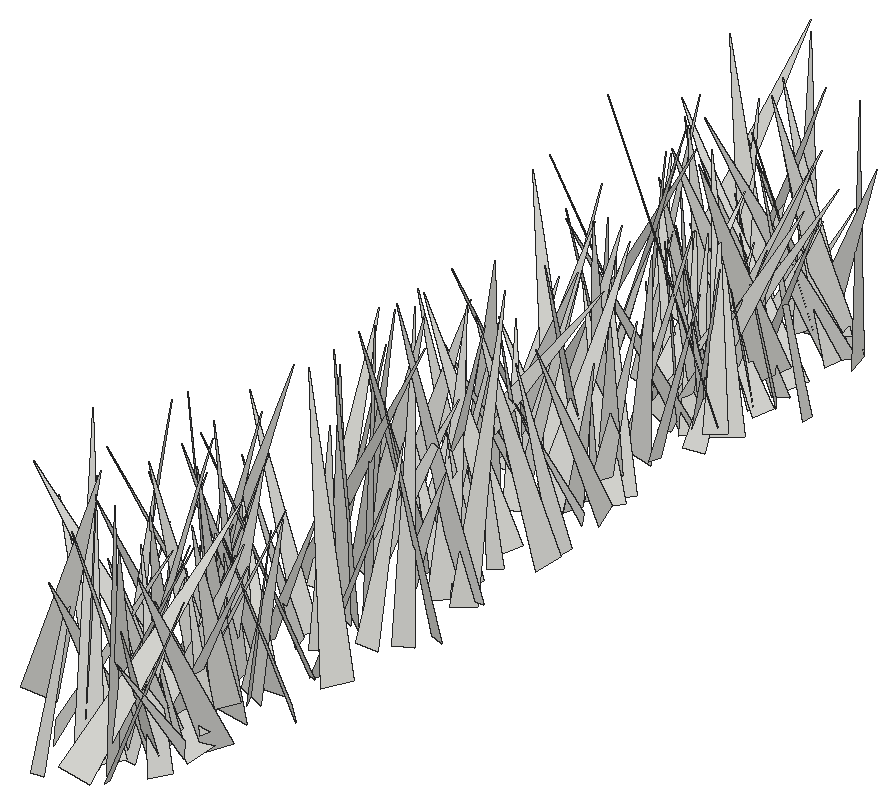
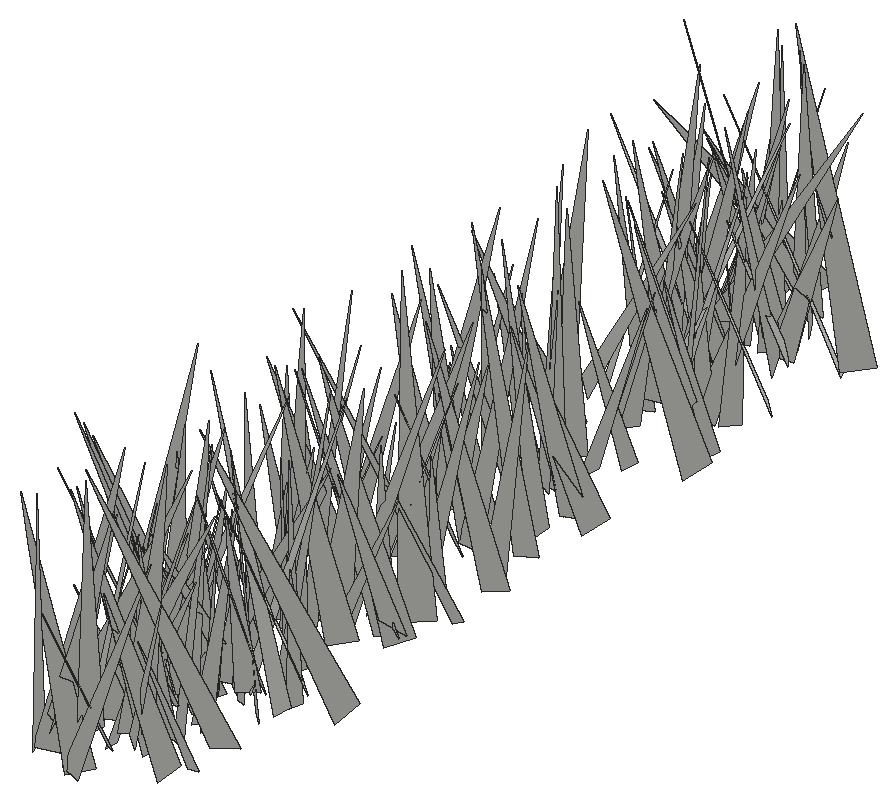
# SketchUp Ruby script. Lengths in inches.
U = 1.inch
M = Sketchup.active_model
def pt(a) = Geom::Point3d.new(a.map { |v| v * U })
def face(e, loops, mat)
  f = e.add_face(loops[0].map { |a| pt(a) })
  loops[1..].each { |l| e.add_face(l.map { |a| pt(a) }).erase! }
  f.material = f.back_material = mat if mat
  f
end
# faces: each face lists its corners as indices into pts; further lists are holes
def faces(e, pts, list, mat = nil) = list.each { |f| face(e, (f[0].is_a?(Array) ? f : [f]).map { |l| l.map { |i| pts[i] } }, mat) }
# xy, xz, yz: faces in a plane at the given z, y or x. An outline is a flat list of corners, or four numbers for a rectangle; further outlines are holes
def ring(l) = l.size == 4 ? [[l[0], l[1]], [l[2], l[1]], [l[2], l[3]], [l[0], l[3]]] : l.each_slice(2).to_a
def flat(e, list, mat, &to3) = list.each { |f| face(e, (f[0].is_a?(Array) ? f : [f]).map { |l| ring(l).map { |u, v| to3.(u, v) } }, mat) }
def xy(e, z, list, mat = nil) = flat(e, list, mat) { |x, y| [x, y, z] }
def xz(e, y, list, mat = nil) = flat(e, list, mat) { |x, z| [x, y, z] }
def yz(e, x, list, mat = nil) = flat(e, list, mat) { |y, z| [x, y, z] }
def lines(e, pts, list) = list.each { |a, b| e.add_line(pt(pts[a]), pt(pts[b])) }
# prism: a flat outline (further loops are holes) pulled along v
def prism(e, loops, v, mat = nil)
  f = face(e, loops, mat); d = Geom::Vector3d.new(v.map { |x| x * U })
  f.pushpull(f.normal.samedirection?(d) ? d.length : -d.length)
end
def box(e, o, s, mat = nil) = prism(e, [[o, [o[0] + s[0], o[1], o[2]], [o[0] + s[0], o[1] + s[1], o[2]], [o[0], o[1] + s[1], o[2]]]], [0, 0, s[2]], mat)
def at(x, y, z, deg = 0) = Geom::Transformation.translation(pt([x, y, z])) * Geom::Transformation.rotation(ORIGIN, Z_AXIS, deg.degrees)
def axes(o, x, y, z) = Geom::Transformation.new([*x, 0, *y, 0, *z, 0, *pt(o).to_a, 1])
def part(name) = M.definitions.add(name)
# library, detail: a bought-in or finely detailed component or shape, given as its bounding box
def library(name, o, s) = part(name).tap { |d| box(d.entities, o, s) }
def detail(e, o, s) = box(e.add_group.entities, o, s)
def put(e, d, t, mat = nil) = e.add_instance(d, t).tap { |i| i.material = mat if mat }
def group(e, t, mat = nil) = e.add_group.tap { |g| g.transformation = t; g.material = mat if mat }.entities
root = M.entities
c1 = part("fur_instance\#9")
p = [[0.8125,0,1.79],[0.67,-0.02,1.48],[0,-0.11,0],[0,0.11,0]]
faces(c1.entities,p,[[0,1,2,3]])
put(root,c1,axes([152.47,140.48,-27.1],[5.88559,1.89129,2.87248],[1.95642,-6.52369,0.2867],[-2.82853,-0.57687,6.17535]))
put(root,c1,axes([150.89,143.3,-28.22],[7.15666,-2.1147,0.99823],[-1.83229,-7.06792,-1.83669],[-1.45298,-1.50292,7.233]))
put(root,c1,axes([153.06,139.34,-27.1],[4.06306,2.1594,0.43468],[1.91332,-3.91175,1.54848],[-1.0914,1.18135,4.33286]))
put(root,c1,axes([152.39,143.6,-28.22],[-1.15105,-5.30671,0.17],[-5.09537,1.15297,1.49093],[1.49242,-0.15644,5.22142]))
put(root,c1,axes([153.89,143.88,-27.1],[-3.33896,-2.6162,0.26799],[-2.1089,2.92233,2.25332],[1.57125,-1.6372,3.59384]))
put(root,c1,axes([148.9,139.44,-28.22],[1.91748,5.33638,0.31642],[5.10909,-1.9283,1.55969],[-1.57297,0.24194,5.4517]))
put(root,c1,axes([152.6,143.37,-28.22],[-5.52316,-3.7636,0.965],[-3.71814,5.60658,0.58551],[1.12752,0.05244,6.65787]))
put(root,c1,axes([149.51,142.25,-27.1],[5.6621,3.46946,2.68851],[3.90579,-5.98471,-0.5026],[-2.00251,-1.86297,6.62147]))
put(root,c1,axes([145.53,143.75,-27.1],[3.43501,-7.39782,1.03394],[-7.28345,-3.06455,2.27067],[1.65774,1.86463,7.83397]))
put(root,c1,axes([148.88,145.0625,-27.1],[3.46816,-3.92613,0.03464],[-3.68547,-3.27126,-1.77763],[-1.35388,-1.15247,4.92774]))
put(root,c1,axes([152.85,144.11,-27.1],[1.51534,-5.37644,0.92666],[-5.31705,-1.67082,-0.99923],[-1.22223,0.60275,5.49581]))
put(root,c1,axes([150.66,140.45,-27.1],[5.57667,1.59527,0.3002],[1.43066,-5.3377,1.78788],[-0.76695,1.64269,5.51794]))
put(root,c1,axes([151.75,140.23,-27.1],[4.07971,3.91858,0.07723],[3.79656,-3.97882,1.32677],[-0.97331,0.90496,5.499]))
put(root,c1,axes([150.89,140.73,-27.1],[-0.59735,8.07244,1.41711],[8.08686,0.34954,1.4177],[-1.33238,-1.49761,7.96939]))
put(root,c1,axes([151.49,138.875,-27.1],[-3.48939,6.7058,0.49493],[5.71017,3.24965,-3.77124],[3.55058,1.36403,6.55144]))
put(root,c1,axes([147.07,143.01,-28.22],[5.77692,4.11347,0.10405],[3.90568,-5.42514,-2.37018],[1.29504,-1.98782,6.68399]))
put(root,c1,axes([153.8,146.52,-28.22],[4.15216,-5.25606,0.30062],[-4.95254,-4.0295,-2.04756],[-1.78575,-1.04593,6.37763]))
put(root,c1,axes([152.77,144.66,-27.1],[-4.67386,-0.0885,1.27111],[0.2568,4.66814,1.26925],[1.24804,-1.29194,4.49909]))
put(root,c1,axes([153.36,142.83,-28.22],[-4.9618,2.41645,1.1014],[2.44275,5.06865,-0.11597],[1.04177,-0.37582,5.51772]))
put(root,c1,axes([151.07,142.99,-28.22],[-0.86303,4.80618,1.97762],[4.83833,1.47497,-1.47315],[1.8976,-1.57489,4.65553]))
put(root,c1,axes([150.88,142.48,-28.22],[-2.13966,5.92839,0.3544],[5.56639,1.87053,2.31645],[-2.07043,-1.09766,5.86157]))
put(root,c1,axes([153.86,143.77,-27.1],[-3.57996,-1.2077,0.30439],[-1.24532,3.48547,-0.8173],[0.0195,0.87192,3.68872]))
put(root,c1,axes([151.1875,142.98,-27.1],[5.81873,5.70667,1.51485],[5.84557,-5.86726,-0.35074],[-0.83073,-1.31442,8.14252]))
put(root,c1,axes([153.53,145.7,-28.22],[-7.78216,2.50032,0.23977],[2.4235,7.26917,2.85602],[-0.66011,-2.78901,7.65877]))
put(root,c1,axes([150.92,143.13,-27.1],[-5.40299,1.91129,1.15946],[1.49374,5.34299,-1.84687],[1.66317,1.41036,5.42535]))
put(root,c1,axes([151.67,144.9375,-28.22],[5.54197,-0.978,0.47716],[-1.05474,-5.437,1.10644],[-0.26776,1.17482,5.51777]))
put(root,c1,axes([153.78,145.83,-27.1],[-3.82053,1.38738,1.41647],[1.59253,3.97908,0.39802],[1.18113,-0.87734,4.0451]))
put(root,c1,axes([152.91,148.23,-27.1],[4.44508,-4.04211,0.97735],[-3.87336,-4.54492,-1.18043],[-1.51359,-0.24009,5.89101]))
put(root,c1,axes([148.67,144.92,-27.1],[3.62249,2.81644,0.55831],[2.6251,-3.61284,1.19278],[-1.16313,0.61769,4.43081]))
put(root,c1,axes([150.79,147.01,-27.1],[1.73127,-4.9492,1.56465],[-4.93445,-1.0575,2.11492],[1.61056,2.08017,4.79781]))
put(root,c1,axes([152.54,149.18,-28.22],[-0.69616,-7.71222,1.47846],[-7.81205,0.83092,0.65597],[0.79755,1.40715,7.71575]))
put(root,c1,axes([151.46,149.03,-28.22],[-6.14349,2.42883,3.06477],[3.31416,6.26335,1.67969],[2.07568,-2.81172,6.38908]))
put(root,c1,axes([150.02,147.22,-28.22],[4.95013,-1.23925,0.4471],[-1.29852,-4.88303,0.8422],[-0.22245,0.9272,5.03291]))
put(root,c1,axes([148.72,145.74,-27.1],[6.05789,3.57549,2.196],[3.19122,-6.43003,1.66595],[-2.72445,0.41853,6.83424]))
put(root,c1,axes([149.47,150.11,-28.22],[0.04578,-6.29285,0.19538],[-6.21134,-0.07706,-1.02644],[-1.02831,0.18529,6.20874]))
put(root,c1,axes([150.63,147.48,-28.22],[6.16739,3.42449,0.19717],[3.4017,-6.05394,-1.25736],[0.441,-1.19388,6.94138]))
put(root,c1,axes([150.01,146.96,-28.22],[2.54415,2.86578,1.34064],[2.68524,-2.86561,1.02977],[-1.67317,-0.2414,3.6912]))
put(root,c1,axes([148.1,149.82,-28.22],[5.5268,-1.95543,1.04999],[-1.67194,-5.52102,-1.48142],[-1.45972,-1.07995,5.67227]))
put(root,c1,axes([151.11,150.91,-27.1],[-5.31992,-4.92486,0.01845],[-4.88394,5.27914,0.91325],[0.63384,-0.65774,7.19179]))
put(root,c1,axes([152.43,146.34,-27.1],[-4.53148,2.02632,0.31118],[1.79338,4.28391,-1.78018],[0.99329,1.50971,4.63371]))
put(root,c1,axes([154.51,151.07,-28.22],[-3.72414,-4.2026,0.59605],[-4.10843,3.76818,0.89886],[1.06672,-0.15915,5.54285]))
put(root,c1,axes([147.7,147.48,-28.22],[3.94824,4.29759,0.4959],[4.2386,-3.97723,0.72087],[-0.86569,0.12707,5.79122]))
put(root,c1,axes([149.59,149.83,-28.22],[-2.80028,2.24736,2.49663],[2.73085,3.4158,-0.01176],[1.95607,-1.55147,3.59055]))
put(root,c1,axes([150.77,150.77,-28.22],[-4.24041,-4.62675,0.86788],[-4.65391,4.29598,0.16351],[0.70788,0.52807,6.27385]))
put(root,c1,axes([153.37,149.22,-27.1],[3.76786,2.01641,1.4087],[2.07515,-3.9894,0.15999],[-1.32064,-0.51569,4.27049]))
put(root,c1,axes([152.01,151.15,-28.22],[-0.32261,-5.78503,1.74562],[-5.69921,0.87225,1.8374],[2.00818,1.5461,5.49497]))
put(root,c1,axes([150.53,150.53,-27.1],[-2.5167,4.57974,3.46384],[4.9953,3.61127,-1.14527],[2.83182,-2.30014,5.09864]))
put(root,c1,axes([152.63,152.1,-28.22],[-1.61608,-6.86234,1.14057],[-6.89566,1.42577,-1.19223],[-0.91789,1.37106,6.94853]))
put(root,c1,axes([151.75,150.65,-27.1],[-6.14594,-1.15799,1.95321],[-1.28361,6.42082,-0.2323],[1.87305,0.60056,6.24977]))
put(root,c1,axes([149.39,151.73,-28.22],[-5.07554,-4.81191,2.50581],[-5.17107,5.32884,-0.24106],[1.64121,1.90882,6.98981]))
put(root,c1,axes([148.09,151.47,-28.22],[5.52496,2.9641,0.73245],[3.00682,-5.54515,-0.24054],[-0.53047,-0.55942,6.26523]))
put(root,c1,axes([151.05,151.78,-27.1],[-1.02276,3.4571,1.0392],[3.60758,1.01767,0.16502],[0.12981,-1.04418,3.60144]))
put(root,c1,axes([154.23,152.73,-27.1],[-4.22462,-4.77942,0.40733],[-4.62488,3.91455,-2.0354],[-1.27248,1.63999,6.04544]))
put(root,c1,axes([147.03,152.47,-28.22],[4.26673,-0.51352,0.23406],[-0.5171,-4.27238,0.05285],[-0.22604,0.08052,4.29719]))
put(root,c1,axes([155.5625,152.92,-27.1],[-6.9298,2.98954,1.57704],[3.02348,7.09089,-0.15622],[1.51094,-0.47802,7.54553]))
put(root,c1,axes([151.59,152.82,-28.22],[-3.84574,2.31871,0.01808],[2.31862,3.84577,-0.02193],[0.02681,0.00945,4.49062]))
put(root,c1,axes([147.67,152.53,-28.22],[6.16496,0.12051,1.82007],[-0.27856,-6.27765,1.3592],[-1.80266,1.38221,6.01447]))
put(root,c1,axes([146.6,154.09,-28.22],[7.47756,-1.51643,1.55812],[-1.8154,-7.42558,1.48539],[-1.19651,1.78955,7.48379]))
put(root,c1,axes([149.3,155.64,-28.22],[4.04534,-0.8517,0.30361],[-0.87788,-4.03293,0.38361],[-0.21657,0.43867,4.11619]))
put(root,c1,axes([150.62,156.42,-28.22],[-4.66141,-1.64687,0.68606],[-1.65466,4.70851,0.06011],[0.66704,0.1713,4.94341]))
put(root,c1,axes([151.94,156.52,-28.22],[2.8988,-5.16102,2.16058],[-5.5292,-3.01461,0.21733],[-0.85564,1.9958,5.91539]))
put(root,c1,axes([153.08,154.35,-28.22],[4.47299,1.54799,0.88013],[1.09405,-4.26651,1.94385],[-1.40498,1.60599,4.31572]))
put(root,c1,axes([150.32,157.37,-28.22],[-5.80532,1.01557,0.17125],[1.00882,5.80466,-0.22508],[0.20737,0.19232,5.88918]))
put(root,c1,axes([151.17,159.58,-28.22],[-3.95013,-6.45103,2.53754],[-6.55598,4.42551,1.04517],[2.25256,1.56763,7.49179]))
put(root,c1,axes([150.49,159.5,-28.22],[-1.6159,-6.90986,2.38073],[-7.13771,2.01606,1.00679],[1.57067,2.05292,7.0245]))
put(root,c1,axes([153.21,158.02,-28.22],[-0.63443,5.02312,1.44392],[5.17666,0.80438,-0.52377],[0.72032,-1.3566,5.03586]))
put(root,c1,axes([155.26,160.57,-28.22],[-3.32572,-4.76152,1.64129],[-5.0351,3.09772,-1.21581],[-0.11678,2.03921,5.67929]))
put(root,c1,axes([146.99,160.98,-28.22],[7.55011,-1.58138,0.22082],[-1.59514,-7.42262,1.38345],[0.0711,1.39915,7.58887]))
put(root,c1,axes([154.46,159.125,-28.22],[1.27817,7.72916,0.81529],[7.27012,-1.48113,2.64386],[-2.74773,-0.32349,7.37453]))
put(root,c1,axes([151.42,160.29,-28.22],[-6.21182,-1.68937,2.27799],[-2.42044,6.01654,-2.13837],[1.47806,2.75267,6.07191]))
put(root,c1,axes([149.16,160.2,-28.22],[5.41894,2.39891,1.8987],[1.67708,-5.5593,2.23748],[-2.55876,1.4367,5.48756]))
put(root,c1,axes([148.27,160.95,-28.22],[-1.26821,6.79621,1.34265],[6.86908,1.41065,-0.65215],[0.89826,-1.19212,6.8827]))
put(root,c1,axes([151,163.73,-28.22],[1.54528,-3.8993,0.59524],[-3.77652,-1.27799,1.43226],[1.13873,1.05307,3.94222]))
put(root,c1,axes([148.56,163.17,-28.22],[7.17764,0.6661,2.04171],[0.73913,-7.45363,-0.1667],[-2.01642,-0.36113,7.20655]))
put(root,c1,axes([149.2,163.07,-28.22],[1.43912,5.66343,2.07225],[5.60003,-0.46439,-2.61988],[2.23794,-2.47985,5.22319]))
put(root,c1,axes([150.27,166.0625,-28.22],[-2.04467,-7.63412,0.65301],[-7.56547,2.11851,1.07815],[1.21235,0.345,7.82931]))
put(root,c1,axes([154.16,164.4,-28.22],[-1.50167,-7.67594,2.08534],[-7.92089,1.24921,-1.10571],[-0.72669,2.24569,7.7429]))
put(root,c1,axes([153.13,163.78,-28.22],[-2.68831,3.38264,1.06218],[3.54497,2.54168,0.8778],[-0.06058,-1.37662,4.23069]))
put(root,c1,axes([147.73,165.14,-28.22],[-0.11111,-7.60969,2.49454],[-7.52897,0.94928,2.56048],[2.72852,2.30953,7.16685]))
put(root,c1,axes([153.17,163.6,-28.22],[-5.91196,3.62871,1.99788],[3.48429,6.23911,-1.02156],[2.24027,-0.12769,6.86114]))
put(root,c1,axes([153.4,165.67,-28.22],[-3.71371,1.13934,1.58672],[1.47505,3.87017,0.67337],[1.28063,-1.15373,3.82574]))
put(root,c1,axes([151.07,165.09,-28.22],[7.16515,0.1083,1.44204],[0.09788,-7.3087,0.06254],[-1.44279,0.042,7.1657]))
put(root,c1,axes([147.72,167.52,-28.22],[4.30794,-3.29071,0.86204],[-3.07513,-4.36194,-1.28347],[-1.45447,-0.52435,5.26686]))
put(root,c1,axes([150.16,165.34,-28.22],[-1.13275,3.97734,1.11963],[3.98013,1.3621,-0.81189],[1.10966,-0.82546,4.05502]))
put(root,c1,axes([154.29,163.72,-28.22],[-6.84761,2.51212,1.52779],[1.98246,6.80446,-2.30302],[2.17135,1.70976,6.92074]))
put(root,c1,axes([153.2,167.39,-28.22],[1.53479,-3.08573,1.52348],[-3.30012,-1.79268,-0.30636],[-0.97569,1.2095,3.43271]))
put(root,c1,axes([152.7,168.94,-28.22],[-5.87282,3.13064,1.60123],[3.47052,5.66214,1.65846],[0.56601,-2.23474,6.44519]))
put(root,c1,axes([154.83,169.21,-28.22],[-6.41083,1.14128,1.69671],[1.48537,6.43646,1.28286],[1.40536,-1.59673,6.38401]))
put(root,c1,axes([146.83,168.46,-28.22],[-0.35143,6.05342,2.99786],[6.31844,1.35633,-1.99808],[2.38924,-2.69649,5.72495]))
put(root,c1,axes([150.78,166.34,-28.22],[2.7978,5.22834,0.27095],[4.99402,-2.75746,1.64099],[-1.57121,0.54549,5.69828]))
put(root,c1,axes([150.33,169.14,-28.22],[-6.00997,1.04438,1.22572],[1.13938,6.10462,0.38513],[1.13796,-0.59647,6.08787]))
put(root,c1,axes([154.74,170.35,-28.22],[-4.85785,0.78834,1.37895],[1.02249,4.94749,0.77364],[1.21552,-1.0112,4.86021]))
put(root,c1,axes([149.15,169.88,-28.22],[-1.47,3.64091,0.87512],[3.73843,1.4809,0.11844],[0.21496,-0.85654,3.92467]))
put(root,c1,axes([147.87,172.93,-28.22],[5.23004,-6.31048,0.45418],[-6.32662,-5.22094,0.31214],[-0.04891,0.54893,8.19012]))
put(root,c1,axes([150.14,173.69,-28.22],[-4.62318,-3.47557,0.41553],[-3.19467,4.47097,1.85217],[1.4305,-1.24775,5.47931]))
put(root,c1,axes([153.46,173.42,-28.22],[-3.32799,-2.15223,0.18164],[-2.02775,3.22824,1.09879],[0.74386,-0.82886,3.80792]))
put(root,c1,axes([154.07,174.3,-28.22],[-5.45284,-1.57742,1.94379],[-0.6971,5.43147,2.45217],[2.40429,-2.00271,5.11943]))
put(root,c1,axes([146.34,171.8125,-28.22],[4.68753,6.76488,0.69054],[6.04009,-3.75687,-4.19721],[3.12373,-2.88717,7.07954]))
put(root,c1,axes([151.12,172.41,-28.22],[1.51862,3.68557,2.40948],[4.21899,-1.94756,0.31991],[-1.2606,-2.07817,3.97332]))
put(root,c1,axes([150.53,172.09,-28.22],[-2.21571,3.96483,0.99922],[4.07213,2.24229,0.13245],[0.36886,-0.93805,4.54001]))
put(root,c1,axes([150.09,175.59,-28.22],[-2.55623,-6.61752,0.06611],[-6.61278,2.55692,0.25211],[0.25899,-0.02922,7.08959]))
put(root,c1,axes([152.57,173.85,-28.22],[4.29298,-1.68508,0.76366],[-1.68331,-4.35833,-0.1541],[-0.76754,0.13347,4.60928]))
put(root,c1,axes([151.63,176.08,-28.22],[-3.16207,-7.07316,1.24758],[-6.76016,3.39142,2.09364],[2.42619,0.2311,7.45956]))
put(root,c1,axes([147.24,174.9375,-28.22],[5.33015,-4.46349,0.382],[-4.4244,-5.15196,1.5366],[0.7024,1.41905,6.78027]))
put(root,c1,axes([151.875,172.56,-28.22],[-2.57926,6.41675,1.59968],[6.21683,2.93816,-1.76197],[2.25493,-0.76079,6.68751]))
put(root,c1,axes([152.59,176.48,-28.22],[2.46673,-5.38252,0.46134],[-5.39282,-2.42347,0.55987],[0.31917,0.65147,5.89431]))
put(root,c1,axes([152.89,175.16,-28.22],[4.40781,-2.35415,1.32075],[-2.57038,-4.43283,0.67704],[-0.82436,1.23418,4.95101]))
put(root,c1,axes([150.21,175.86,-28.22],[-3.99734,1.08155,0.32432],[1.12476,3.91891,0.79421],[0.09918,-0.85212,4.0642]))
put(root,c1,axes([149.96,173.3125,-28.22],[3.95249,6.61953,0.92655],[6.54498,-4.05132,1.02412],[-1.35642,-0.25967,7.64143]))
put(root,c1,axes([148.07,174.91,-28.22],[0.74046,6.81709,2.01452],[6.9144,-0.22063,-1.79488],[1.64984,-2.13492,6.61811]))
put(root,c1,axes([151.66,177.2,-28.22],[-0.40221,-7.56998,1.93164],[-7.73436,0.65878,0.97125],[1.10251,1.85984,7.51818]))
put(root,c1,axes([147.57,174.8,-28.22],[-1.59343,4.55905,1.08338],[4.45907,1.82697,-1.12985],[1.44061,-0.61229,4.69546]))
put(root,c1,axes([153.75,175.3,-28.22],[-4.34264,3.05124,0.46122],[3.07623,4.34339,0.23041],[0.24406,-0.45414,5.3024]))
put(root,c1,axes([150.76,175.375,-28.22],[2.27452,-5.56414,4.58515],[-6.58849,-3.55674,-1.04785],[-2.92831,3.68058,5.91904]))
put(root,c1,axes([149.27,176.61,-28.22],[3.87683,-5.48097,2.21285],[-5.90731,-3.50163,1.67625],[0.20355,2.76859,6.50085]))
put(root,c1,axes([153.72,176.27,-28.22],[-4.80614,1.67739,0.07303],[1.63862,4.73444,-0.90443],[0.36591,0.83033,5.00945]))
put(root,c1,axes([151.96,179.47,-28.22],[0.10364,-5.95888,1.80759],[-6.13378,0.21397,1.05707],[1.07352,1.79787,5.86529]))
put(root,c1,axes([151.13,178.35,-28.22],[-4.67336,-1.61213,2.14084],[-2.03116,4.93814,-0.71533],[1.7483,1.42769,4.89159]))
put(root,c1,axes([148.8,181.72,-28.22],[-3.51133,-6.12863,1.17286],[-5.90116,3.69891,1.66117],[2.0278,0.152,6.86513]))
put(root,c1,axes([152.58,179.78,-28.22],[4.041,0.55824,1.1889],[0.26805,-4.11576,1.02147],[-1.28579,0.89645,3.94942]))
put(root,c1,axes([150.72,180.12,-28.22],[-2.72966,-3.54913,3.67888],[-4.47058,3.67982,0.23296],[2.47878,2.72838,4.47136]))
put(root,c1,axes([149.2,179.91,-28.22],[-3.18847,2.06393,0.29466],[1.98964,3.17316,-0.69666],[0.62286,0.42918,3.73374]))
put(root,c1,axes([152.16,182.79,-28.22],[-1.24481,-6.10899,0.55091],[-5.80958,0.99391,-2.10566],[-1.96776,0.93016,5.86818]))
put(root,c1,axes([148.79,184.14,-27.1],[-4.50054,-5.78959,0.45114],[-5.68851,4.51005,1.13049],[1.1678,-0.3432,7.24542]))
put(root,c1,axes([147.29,182.56,-28.22],[5.69502,0.05498,1.49404],[0.36012,-5.7612,-1.16071],[-1.45103,-1.21405,5.57575]))
put(root,c1,axes([152.78,183.46,-28.22],[3.64038,-1.44849,0.64201],[-1.22649,-3.59476,-1.15586],[-1.003,-0.8615,3.74359]))
put(root,c1,axes([152.82,182.28,-28.22],[4.61454,1.12705,1.27743],[1.23829,-4.75228,-0.2803],[-1.16993,-0.58453,4.7419]))
put(root,c1,axes([154.44,181.86,-27.1],[-3.13208,3.88614,1.48189],[4.03166,3.29255,-0.11327],[1.02167,-1.07935,4.98991]))
put(root,c1,axes([152.23,183.45,-27.1],[0.17037,-4.40384,1.04145],[-4.5148,-0.2364,-0.26107],[-0.30825,1.02847,4.3994]))
put(root,c1,axes([153.88,182.68,-27.1],[-6.31099,-5.2237,1.0112],[-5.28027,5.95593,-2.18722],[-0.65451,2.31907,7.89505]))
put(root,c1,axes([149.46,183.75,-28.22],[-1.86728,-3.21645,1.13397],[-3.16749,2.11482,0.78275],[1.26429,0.54787,3.63587]))
put(root,c1,axes([144.96,181.61,-28.22],[7.82793,-0.68601,0.13891],[-0.69946,-7.6099,1.83483],[0.02566,1.8399,7.64072]))
put(root,c1,axes([150.87,183.62,-28.22],[-3.54566,-2.66431,1.6705],[-2.78653,3.82874,0.19209],[1.45754,0.83849,4.43096]))
put(root,c1,axes([149.875,183.02,-28.22],[1.07989,-3.22676,1.49499],[-3.22529,-0.23045,1.83235],[1.49815,1.82977,2.86716]))
put(root,c1,axes([148.21,180.68,-28.22],[4.01654,5.38759,0.39242],[5.219,-3.99648,1.45013],[-1.3936,0.56102,6.56169]))
put(root,c1,axes([151.22,182.16,-28.22],[3.96425,-0.56902,0.64503],[-0.79665,-3.57598,1.74151],[-0.32433,1.82859,3.60641]))
put(root,c1,axes([146.15,184.83,-27.1],[7.97506,1.59703,0.67128],[1.71117,-7.75527,-1.87893],[-0.27022,-1.97686,7.91339]))
put(root,c1,axes([152.8125,184,-28.22],[-4.28874,-2.62611,1.19653],[-2.76089,4.3576,-0.33198],[0.84,0.91449,5.01792]))
put(root,c1,axes([152.33,182.58,-28.22],[-4.55116,2.07867,0.64916],[1.93391,4.54938,-1.00919],[1.00113,0.66152,4.90056]))
put(root,c1,axes([153.82,183.49,-28.22],[-4.3858,5.26104,2.02142],[5.54364,4.48874,0.34523],[1.01623,-1.78118,6.84066]))
put(root,c1,axes([153.4375,181.53,-28.22],[-3.94545,3.07895,0.18102],[2.74281,3.63702,-2.08047],[1.41057,1.53994,4.55172]))
put(root,c1,axes([153.12,187.67,-27.1],[6.488,-4.94571,0.82766],[-4.48999,-6.33233,-2.64212],[-2.23271,-1.63731,7.71838]))
put(root,c1,axes([148.02,184.35,-28.22],[-4.08433,-4.26667,3.28401],[-4.58243,4.91876,0.69141],[2.82675,1.80893,5.86585]))
put(root,c1,axes([150.02,184.33,-27.1],[-1.79664,3.17113,0.9039],[3.29721,1.71578,0.53432],[-0.03822,-1.04932,3.60534]))
put(root,c1,axes([151.32,184.23,-27.1],[-2.54986,2.80817,1.27437],[2.87177,2.76487,-0.34653],[1.12374,-0.69377,3.77724]))
put(root,c1,axes([150.64,184.32,-28.22],[3.61026,-5.57217,1.81458],[-5.57053,-2.60139,3.09478],[1.81959,3.09184,5.87413]))
put(root,c1,axes([152.62,186.84,-28.22],[-2.708,-3.38854,1.07596],[-2.8715,2.88211,1.84961],[2.09627,-0.42942,3.92357]))
put(root,c1,axes([154.86,185.72,-27.1],[-3.48684,-2.54111,1.02639],[-2.66037,3.53733,-0.28017],[0.65812,0.83597,4.30544]))
put(root,c1,axes([148.54,184.39,-27.1],[-2.22109,4.73282,1.14399],[4.81333,2.32397,-0.26934],[0.73496,-0.91711,5.22114]))
put(root,c1,axes([150.7,186.4375,-27.1],[3.54462,-5.56954,2.15269],[-5.7416,-3.86654,-0.54956],[-1.63946,1.49942,6.57891]))
put(root,c1,axes([149.64,183.7,-27.1],[-1.38897,4.86037,0.26759],[4.61521,1.40338,-1.53442],[1.54748,0.17706,4.81643]))
put(root,c1,axes([151.85,185.09,-27.1],[6.12264,-2.56902,1.18593],[-2.80714,-5.86992,1.77677],[-0.35534,2.10644,6.39763]))
put(root,c1,axes([153.71,186.23,-28.22],[-4.37284,2.10544,0.41102],[2.13916,4.20984,1.19366],[-0.16073,-1.25217,4.70423]))
put(root,c1,axes([151.7,188.4,-27.1],[4.33462,-5.23656,1.50263],[-4.77333,-4.57611,-2.17783],[-2.62578,-0.3257,6.43953]))
put(root,c1,axes([148.57,183.42,-27.1],[3.46655,5.88623,0.70358],[5.62008,-3.5225,1.77941],[-1.8861,0.32244,6.59533]))
put(root,c1,axes([150.51,186.68,-28.22],[3.81482,2.67004,0.71919],[2.75746,-3.58156,-1.32965],[0.20681,-1.49748,4.4625]))
put(root,c1,axes([148.3,187.99,-27.1],[-4.48343,0.78051,2.64752],[1.64873,4.80743,1.37477],[2.21365,-1.99978,4.33824]))
put(root,c1,axes([150.09,185.98,-28.22],[4.07945,6.65627,1.20942],[6.56454,-3.55321,-2.58689],[1.63565,-2.3408,7.36585]))
put(root,c1,axes([149.32,186.53,-28.22],[-4.30965,-1.39305,1.63599],[-1.58025,4.5392,-0.29767],[1.45598,0.80324,4.51941]))
put(root,c1,axes([153.16,186.55,-28.22],[-3.62089,2.64212,0.01483],[2.58278,3.53416,0.96476],[-0.55698,-0.78788,4.37731]))
put(root,c1,axes([153.42,187.91,-28.22],[-0.61117,-4.98438,1.28841],[-4.9544,0.21679,-1.51148],[-1.3993,1.40945,4.78884]))
put(root,c1,axes([149.22,188.6,-28.22],[-4.05006,-5.82532,2.03849],[-5.82326,4.4146,1.04584],[2.04438,1.03428,7.01738]))
put(root,c1,axes([150.24,187.43,-27.1],[4.10846,4.74791,0.21399],[4.46685,-3.7608,-2.31765],[1.62348,-1.66782,5.83529]))
put(root,c1,axes([151.43,188.86,-28.22],[0.99148,-3.49866,0.36174],[-3.47594,-0.91715,0.65665],[0.53788,0.52224,3.57665]))
put(root,c1,axes([151.82,188.46,-27.1],[5.27208,0.02621,0.0042],[0.02652,-5.23568,-0.61848],[-0.0011,-0.61849,5.23574]))
put(root,c1,axes([155.62,187.05,-28.22],[-5.8174,-1.77979,0.63377],[-1.88895,5.44209,-2.05595],[-0.03436,2.15114,5.72563]))
put(root,c1,axes([151.52,190.6,-28.22],[-5.8383,-2.13052,1.19785],[-1.77007,5.82456,1.73238],[1.68547,-1.263,5.96857]))
put(root,c1,axes([151.78,187.68,-28.22],[-2.40389,3.30252,0.08348],[3.28439,2.37806,0.4999],[-0.35549,-0.36124,4.05406]))
put(root,c1,axes([153.32,188.85,-28.22],[-6.06762,4.08752,0.30456],[4.00596,5.79855,1.98636],[-0.86766,-1.81261,7.04117]))
put(root,c1,axes([151.16,189.73,-27.1],[-2.98198,-2.20876,0.85448],[-2.34628,2.94214,-0.58291],[0.32208,0.98295,3.66484]))
put(root,c1,axes([153.41,192.27,-28.22],[1.64942,-7.33453,1.1804],[-6.83961,-1.97125,-2.69132],[-2.89974,0.47759,7.01946]))
put(root,c1,axes([150.27,189.01,-28.22],[0.79551,4.29487,0.6755],[4.10301,-0.51451,-1.56067],[1.4379,-0.90797,4.07959]))
put(root,c1,axes([150.0625,188.37,-28.22],[-0.0106,6.43156,0.96228],[6.47441,-0.07994,0.60561],[-0.61077,-0.95901,6.403]))
put(root,c1,axes([151.24,192.81,-27.1],[-4.09949,-5.26965,1.04192],[-4.89422,4.20438,2.00758],[2.21389,-0.46331,6.36747]))
put(root,c1,axes([150.1,190.59,-27.1],[-5.03128,5.10175,2.45438],[5.52933,5.13327,0.66454],[1.21582,-2.23324,7.13442]))
put(root,c1,axes([147.2,190.01,-28.22],[0.85166,3.52496,0.51911],[3.494,-0.72175,-0.83136],[0.69768,-0.68839,3.5298]))
put(root,c1,axes([153.375,192.67,-28.22],[3.93699,-6.31061,2.13001],[-6.14082,-4.39732,-1.67764],[-2.57895,0.83692,7.24632]))
put(root,c1,axes([149.71,189.84,-28.22],[4.12915,-1.39251,2.24683],[-2.1688,-4.1671,1.40312],[-1.51116,2.17563,4.12556]))
put(root,c1,axes([153.36,192.1,-28.22],[-5.54142,2.04017,2.02802],[2.50487,5.58649,1.22443],[1.41448,-1.90035,5.77671]))
put(root,c1,axes([146.08,189.1,-27.1],[0.28527,8.21503,1.11931],[7.94931,0.04717,-2.37217],[2.35543,-1.15413,7.87026]))
put(root,c1,axes([147.82,190.98,-28.22],[7.40622,-0.19557,0.80001],[-0.28757,-7.3972,0.85392],[-0.77173,0.87956,7.35943]))
put(root,c1,axes([149.73,191.3,-27.1],[1.87721,3.55983,2.07479],[3.45548,-2.60202,1.33802],[-2.2443,-1.02868,3.79553]))
put(root,c1,axes([151.11,193.37,-28.22],[3.81645,-5.44593,0.15233],[-5.28758,-3.65777,1.70554],[1.31259,1.09964,6.42764]))
put(root,c1,axes([153.16,192.32,-27.1],[1.40362,-5.52471,3.15038],[-5.88186,-2.35471,-1.50878],[-2.41887,2.51999,5.49692]))
put(root,c1,axes([151.34,193.77,-28.22],[-1.836,-5.36618,0.72675],[-5.38286,1.72484,-0.86298],[-0.59066,0.96126,5.60554]))
put(root,c1,axes([151.72,191.86,-27.1],[-6.82221,1.72842,2.33339],[1.55801,7.20655,-0.7829],[2.45045,0.23004,6.99407]))
put(root,c1,axes([154.18,192.52,-28.22],[5.88559,1.89129,2.87248],[1.95642,-6.52369,0.2867],[-2.82853,-0.57687,6.17535]))
put(root,c1,axes([150.13,192.36,-27.1],[2.36408,2.77163,0.06713],[2.67068,-2.25294,-1.03299],[0.74428,-0.71945,3.49339]))
